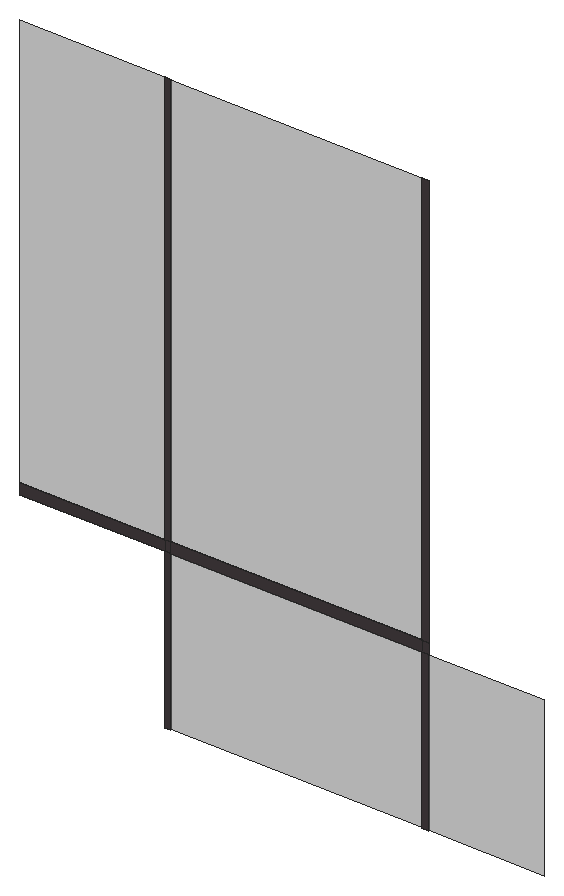
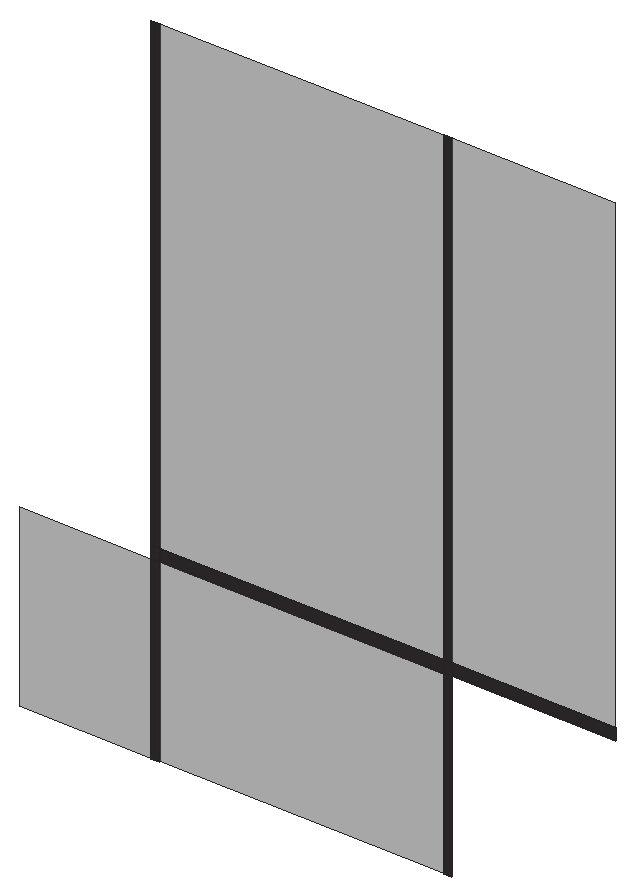
# SketchUp Ruby script. Lengths in inches.
U = 1.inch
M = Sketchup.active_model
def pt(a) = Geom::Point3d.new(a.map { |v| v * U })
def face(e, loops, mat)
  f = e.add_face(loops[0].map { |a| pt(a) })
  loops[1..].each { |l| e.add_face(l.map { |a| pt(a) }).erase! }
  f.material = f.back_material = mat if mat
  f
end
# faces: each face lists its corners as indices into pts; further lists are holes
def faces(e, pts, list, mat = nil) = list.each { |f| face(e, (f[0].is_a?(Array) ? f : [f]).map { |l| l.map { |i| pts[i] } }, mat) }
# xy, xz, yz: faces in a plane at the given z, y or x. An outline is a flat list of corners, or four numbers for a rectangle; further outlines are holes
def ring(l) = l.size == 4 ? [[l[0], l[1]], [l[2], l[1]], [l[2], l[3]], [l[0], l[3]]] : l.each_slice(2).to_a
def flat(e, list, mat, &to3) = list.each { |f| face(e, (f[0].is_a?(Array) ? f : [f]).map { |l| ring(l).map { |u, v| to3.(u, v) } }, mat) }
def xy(e, z, list, mat = nil) = flat(e, list, mat) { |x, y| [x, y, z] }
def xz(e, y, list, mat = nil) = flat(e, list, mat) { |x, z| [x, y, z] }
def yz(e, x, list, mat = nil) = flat(e, list, mat) { |y, z| [x, y, z] }
def lines(e, pts, list) = list.each { |a, b| e.add_line(pt(pts[a]), pt(pts[b])) }
# prism: a flat outline (further loops are holes) pulled along v
def prism(e, loops, v, mat = nil)
  f = face(e, loops, mat); d = Geom::Vector3d.new(v.map { |x| x * U })
  f.pushpull(f.normal.samedirection?(d) ? d.length : -d.length)
end
def box(e, o, s, mat = nil) = prism(e, [[o, [o[0] + s[0], o[1], o[2]], [o[0] + s[0], o[1] + s[1], o[2]], [o[0], o[1] + s[1], o[2]]]], [0, 0, s[2]], mat)
def at(x, y, z, deg = 0) = Geom::Transformation.translation(pt([x, y, z])) * Geom::Transformation.rotation(ORIGIN, Z_AXIS, deg.degrees)
def axes(o, x, y, z) = Geom::Transformation.new([*x, 0, *y, 0, *z, 0, *pt(o).to_a, 1])
def part(name) = M.definitions.add(name)
# library, detail: a bought-in or finely detailed component or shape, given as its bounding box
def library(name, o, s) = part(name).tap { |d| box(d.entities, o, s) }
def detail(e, o, s) = box(e.add_group.entities, o, s)
def put(e, d, t, mat = nil) = e.add_instance(d, t).tap { |i| i.material = mat if mat }
def group(e, t, mat = nil) = e.add_group.tap { |g| g.transformation = t; g.material = mat if mat }.entities
root = M.entities
M.materials.add("[Asphalt New]").color = [67, 60, 62]
M.materials.add("[Translucent Glass Gray]").color = [128, 128, 128]
M.materials["[Translucent Glass Gray]"].alpha = 0.5
xz(root,304.24,[[208.29,4.22,210.23,52.25],[286.57,4.22,288.77,52.25],[164.29,52.25,208.29,55.45],[208.29,52.25,210.23,55.45],[210.23,52.25,286.57,55.45],
  [286.57,52.25,288.77,55.45],[208.29,55.45,210.23,181.51],[286.57,55.45,288.77,181.51]],"[Asphalt New]")
xz(root,304.24,[[210.23,4.22,286.57,52.25],[288.77,4.22,323.93,52.25],[164.29,55.45,208.29,181.51],[210.23,55.45,286.57,181.51]],"[Translucent Glass Gray]")
